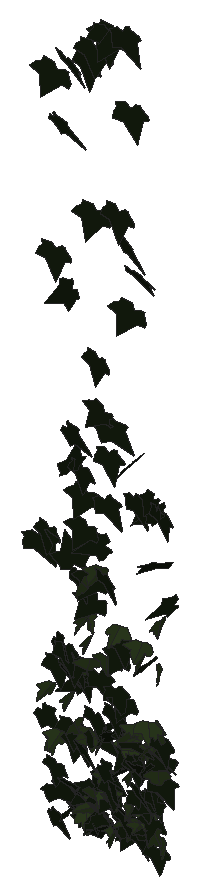
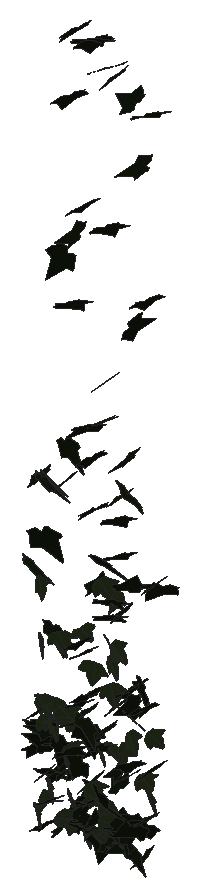
# SketchUp Ruby script. Lengths in inches.
U = 1.inch
M = Sketchup.active_model
def pt(a) = Geom::Point3d.new(a.map { |v| v * U })
def face(e, loops, mat)
  f = e.add_face(loops[0].map { |a| pt(a) })
  loops[1..].each { |l| e.add_face(l.map { |a| pt(a) }).erase! }
  f.material = f.back_material = mat if mat
  f
end
# faces: each face lists its corners as indices into pts; further lists are holes
def faces(e, pts, list, mat = nil) = list.each { |f| face(e, (f[0].is_a?(Array) ? f : [f]).map { |l| l.map { |i| pts[i] } }, mat) }
# xy, xz, yz: faces in a plane at the given z, y or x. An outline is a flat list of corners, or four numbers for a rectangle; further outlines are holes
def ring(l) = l.size == 4 ? [[l[0], l[1]], [l[2], l[1]], [l[2], l[3]], [l[0], l[3]]] : l.each_slice(2).to_a
def flat(e, list, mat, &to3) = list.each { |f| face(e, (f[0].is_a?(Array) ? f : [f]).map { |l| ring(l).map { |u, v| to3.(u, v) } }, mat) }
def xy(e, z, list, mat = nil) = flat(e, list, mat) { |x, y| [x, y, z] }
def xz(e, y, list, mat = nil) = flat(e, list, mat) { |x, z| [x, y, z] }
def yz(e, x, list, mat = nil) = flat(e, list, mat) { |y, z| [x, y, z] }
def lines(e, pts, list) = list.each { |a, b| e.add_line(pt(pts[a]), pt(pts[b])) }
# prism: a flat outline (further loops are holes) pulled along v
def prism(e, loops, v, mat = nil)
  f = face(e, loops, mat); d = Geom::Vector3d.new(v.map { |x| x * U })
  f.pushpull(f.normal.samedirection?(d) ? d.length : -d.length)
end
def box(e, o, s, mat = nil) = prism(e, [[o, [o[0] + s[0], o[1], o[2]], [o[0] + s[0], o[1] + s[1], o[2]], [o[0], o[1] + s[1], o[2]]]], [0, 0, s[2]], mat)
def at(x, y, z, deg = 0) = Geom::Transformation.translation(pt([x, y, z])) * Geom::Transformation.rotation(ORIGIN, Z_AXIS, deg.degrees)
def axes(o, x, y, z) = Geom::Transformation.new([*x, 0, *y, 0, *z, 0, *pt(o).to_a, 1])
def part(name) = M.definitions.add(name)
# library, detail: a bought-in or finely detailed component or shape, given as its bounding box
def library(name, o, s) = part(name).tap { |d| box(d.entities, o, s) }
def detail(e, o, s) = box(e.add_group.entities, o, s)
def put(e, d, t, mat = nil) = e.add_instance(d, t).tap { |i| i.material = mat if mat }
def group(e, t, mat = nil) = e.add_group.tap { |g| g.transformation = t; g.material = mat if mat }.entities
root = M.entities
M.materials.add("1026 AP 7946 SUNNY SIDE UP").color = [254, 231, 186]
M.materials.add("efeu1").color = [18, 25, 13]
M.materials.add("efeu2").color = [43, 57, 29]
c1 = part("ivyleaf_10")
p = [[0,0.5,-0.03],[-0.0625,2.02,-0.43],[-0.19,2.01,-0.46],[-0.54,1.05,-0.29],[-0.52,0.625,-0.18],[-0.83,0.76,-0.28],
  [-1.16,0.64,-0.33],[-1.15,0.33,-0.24],[-0.77,-0.39,0.02],[-0.3,-0.51,0.16],[0.04,-0.48,0.23],[-0.02,2.01,-0.4375],
  [-0.06,2.01,-0.43],[0.04,-0.49,0.23],[0.67,-0.49,0.14],[1.38,0.36,-0.2],[1.375,0.51,-0.24],[0.81,0.65,-0.19],
  [0.62,0.59,-0.15],[0.6,1.09,-0.28],[0.5,1.23,-0.31]]
faces(c1.entities,p,[[0,1,2,3,4,5,6,7,8,9,10],[11,12,0,13,14,15,16,17,18,19,20]],"efeu2")
c2 = part("ivyleaf_9")
p = [[1.54,2.16,1.25],[1.36,2.04,1.19],[-0.21,0.99,0.68],[-0.71,1.11,0.82],[-0.85,0.86,0.67],[-0.8,0.17,0.21],
  [-0.9,-0.01,0.1],[-0.67,-0.16,-0.02],[-0.08,-0.08,-0.05],[-0.03,-0.6,-0.4],[0.65,-0.88,-0.66],[0.83,-0.6,-0.49],
  [1.29,-0.42,-0.43],[1.8125,-0.07,-0.26],[1.21,0.44,0.15]]
faces(c2.entities,p,[[0,1,2,3,4,5,6,7,8,9,10,11,12,13,14]],"efeu1")
put(root,c1,axes([134.13,212.53,294.28],[0.33293,-0.26195,-0.18887],[-0.15797,0.15237,-0.34573],[0.47588,0.23384,0.01737]),"1026 AP 7946 SUNNY SIDE UP")
put(root,c2,axes([133.74,212.17,304.24],[-0.13472,-0.32165,-0.27255],[0.20303,0.23434,-0.33756],[0.62068,-0.14647,0.05126]),"1026 AP 7946 SUNNY SIDE UP")
put(root,c2,axes([133.88,212.625,304.42],[-0.05844,-0.37294,0.13765],[-0.03565,-0.13411,-0.38678],[0.62303,-0.04265,-0.00922]),"1026 AP 7946 SUNNY SIDE UP")
put(root,c1,axes([134.12,212.36,297.02],[-0.10301,-0.29039,0.23968],[-0.02573,-0.23542,-0.30668],[0.58614,-0.06137,0.02866]),"1026 AP 7946 SUNNY SIDE UP")
put(root,c2,axes([133.82,212.36,295.7],[0.26681,-0.28497,-0.23819],[-0.09029,0.2292,-0.33545],[0.56828,0.17021,0.05853]),"1026 AP 7946 SUNNY SIDE UP")
put(root,c2,axes([134.19,212.69,318.03],[-0.1405,-0.4347,0.0012],[0.00417,-0.00426,-0.4572],[0.68354,-0.08933,0.00304]),"1026 AP 7946 SUNNY SIDE UP")
put(root,c2,axes([134.34,212.52,326.82],[-0.41289,-0.37471,0.12809],[0.01519,-0.15783,-0.46204],[0.62165,-0.24502,0.09636]),"1026 AP 7946 SUNNY SIDE UP")
put(root,c2,axes([134.22,212.72,293.07],[-0.08881,-0.32549,0.15097],[0.04328,-0.15374,-0.33751],[0.56082,-0.03968,0.04996]),"1026 AP 7946 SUNNY SIDE UP")
put(root,c1,axes([134.59,212.38,294.82],[-0.24139,-0.27422,0.22648],[0.0221,-0.24606,-0.30537],[0.55374,-0.10972,0.11092]),"1026 AP 7946 SUNNY SIDE UP")
put(root,c2,axes([134.48,212.51,298.29],[-0.08486,-0.39007,-0.02198],[0.0001,0.0193,-0.40555],[0.61408,-0.0539,-0.00297]),"1026 AP 7946 SUNNY SIDE UP")
put(root,c2,axes([134.35,212.6,299.22],[0.02918,-0.12609,-0.38308],[0.60824,-0.05416,0.03857],[-0.09961,-0.36764,0.12325]),"1026 AP 7946 SUNNY SIDE UP")
put(root,c2,axes([134.34,212.58,324.43],[0.52513,-0.31138,-0.06126],[0.01397,0.09304,-0.46371],[0.49775,0.32589,0.07765]),"1026 AP 7946 SUNNY SIDE UP")
put(root,c2,axes([134.53,212.125,291.1],[0.32327,-0.27561,-0.11867],[-0.10007,0.09427,-0.35363],[0.45795,0.21516,0.00649]),"1026 AP 7946 SUNNY SIDE UP")
put(root,c2,axes([135.16,212.43,291.24],[-0.21083,0.3254,-0.01468],[-0.00983,-0.01997,-0.36243],[-0.5122,-0.13356,0.013]),"1026 AP 7946 SUNNY SIDE UP")
put(root,c2,axes([134.62,212.15,292.4375],[0.03625,-0.139,-0.36574],[0.18005,0.34096,-0.12817],[0.57061,-0.09876,0.06368]),"1026 AP 7946 SUNNY SIDE UP")
put(root,c1,axes([135.04,212.625,296.77],[-0.00007,-0.38183,0.03941],[-0.00016,-0.04043,-0.39359],[0.60374,-0.00006,-0.0001]),"1026 AP 7946 SUNNY SIDE UP")
put(root,c2,axes([135.05,212.62,316.4375],[0.00082,-0.21928,-0.43947],[0.28433,-0.39372,0.20703],[-0.69667,-0.16094,0.08398]),"1026 AP 7946 SUNNY SIDE UP")
put(root,c2,axes([134.74,212.4,292.5],[0.56784,0.02559,0.08434],[0.13176,-0.03258,-0.37115],[-0.02776,0.36882,-0.03645]),"1026 AP 7946 SUNNY SIDE UP")
put(root,c2,axes([134.73,212.79,327.375],[0.22262,-0.37505,0.24704],[0.18751,-0.21279,-0.41298],[0.67626,0.18246,0.03319]),"1026 AP 7946 SUNNY SIDE UP")
put(root,c2,axes([135,212.37,299.14],[0.02752,-0.39373,-0.01249],[-0.00676,0.0097,-0.40594],[0.61926,0.0176,-0.00388]),"1026 AP 7946 SUNNY SIDE UP")
put(root,c2,axes([135.4,212.24,308.1],[-0.50944,0.28383,-0.19066],[-0.18303,0.14961,0.44332],[0.50185,0.34269,-0.03187]),"1026 AP 7946 SUNNY SIDE UP")
put(root,c2,axes([135.17,212.625,295.42],[-0.17406,-0.35467,-0.0606],[0.03547,0.05247,-0.38241],[0.56368,-0.11282,0.00535]),"1026 AP 7946 SUNNY SIDE UP")
put(root,c2,axes([135.53,212.24,303.56],[-0.54205,-0.18855,0.16931],[0.20464,0.1059,0.40437],[-0.33716,0.3674,-0.02678]),"1026 AP 7946 SUNNY SIDE UP")
put(root,c2,axes([134.98,212.29,298.13],[0.51508,-0.19503,0.03846],[0.02793,-0.04508,-0.39183],[0.31131,0.32673,-0.02848]),"1026 AP 7946 SUNNY SIDE UP")
put(root,c2,axes([135.33,212.66,294.73],[-0.11052,-0.34686,0.12552],[0.00577,-0.1267,-0.36426],[0.57907,-0.06494,0.02758]),"1026 AP 7946 SUNNY SIDE UP")
put(root,c2,axes([135.87,212.41,297.84],[-0.54011,0.17301,0.01063],[-0.03987,-0.02969,-0.39446],[-0.26951,-0.34233,0.03705]),"1026 AP 7946 SUNNY SIDE UP")
put(root,c2,axes([135.22,212.48,291.52],[0.49824,-0.18281,0.01197],[0.01835,-0.0051,-0.37689],[0.28755,0.31708,0.00331]),"1026 AP 7946 SUNNY SIDE UP")
put(root,c2,axes([135.45,212.4375,298.71],[-0.11702,-0.38131,0.0361],[-0.00021,-0.03788,-0.40039],[0.60242,-0.07408,0.00688]),"1026 AP 7946 SUNNY SIDE UP")
put(root,c2,axes([135.33,212.16,309.95],[0.40059,-0.29519,-0.18227],[-0.10396,0.17197,-0.3964],[0.52969,0.257,0.06005]),"1026 AP 7946 SUNNY SIDE UP")
put(root,c2,axes([135.39,212.76,302.66],[0.12527,-0.38162,0.07901],[0.00832,-0.07942,-0.40193],[0.61268,0.0791,-0.01069]),"1026 AP 7946 SUNNY SIDE UP")
put(root,c1,axes([135.71,212.12,295.8125],[-0.11454,-0.3205,-0.20139],[0.11258,0.18173,-0.33652],[0.57795,-0.09892,0.02564]),"1026 AP 7946 SUNNY SIDE UP")
put(root,c1,axes([135.83,212.62,300.75],[0.02841,-0.36397,0.1611],[-0.0157,-0.15898,-0.37598],[0.62399,0.01257,-0.0168]),"1026 AP 7946 SUNNY SIDE UP")
put(root,c2,axes([135.54,212.73,294.27],[0.04237,-0.25488,0.26857],[0.15172,-0.24858,-0.26066],[0.55454,0.08749,0.0508]),"1026 AP 7946 SUNNY SIDE UP")
put(root,c2,axes([135.84,212.68,305.18],[-0.33757,-0.32453,0.11841],[-0.02098,-0.12964,-0.39717],[0.54193,-0.20717,0.05838]),"1026 AP 7946 SUNNY SIDE UP")
put(root,c2,axes([135.7,212.61,307.96],[-0.038,-0.37972,0.16198],[0.02841,-0.16048,-0.392],[0.64691,-0.01526,0.02673]),"1026 AP 7946 SUNNY SIDE UP")
put(root,c2,axes([135.95,212.58,306.87],[-0.36768,-0.3281,0.05341],[-0.00843,-0.06193,-0.41417],[0.5227,-0.23179,0.03089]),"1026 AP 7946 SUNNY SIDE UP")
put(root,c1,axes([136.0625,212.64,298.74],[-0.37255,-0.30325,0.0503],[-0.01619,-0.05595,-0.39586],[0.48314,-0.23571,0.02552]),"1026 AP 7946 SUNNY SIDE UP")
put(root,c2,axes([135.78,212.65,297.97],[0.0469,-0.37594,0.07841],[0.01126,-0.07792,-0.38896],[0.60369,0.03066,0.00117]),"1026 AP 7946 SUNNY SIDE UP")
put(root,c2,axes([136.4,212.21,291.54],[-0.28359,0.29837,0.11667],[-0.13408,0.0783,-0.35729],[-0.48259,-0.19709,0.03071]),"1026 AP 7946 SUNNY SIDE UP")
put(root,c1,axes([136.16,212.53,299.97],[0.05495,-0.38936,0.04866],[0.00257,-0.04949,-0.403],[0.61714,0.03487,-0.00266]),"1026 AP 7946 SUNNY SIDE UP")
put(root,c2,axes([135.83,212.27,294.79],[0.3657,-0.29299,0.00758],[-0.01187,-0.0175,-0.38509],[0.46077,0.23209,-0.01594]),"1026 AP 7946 SUNNY SIDE UP")
put(root,c2,axes([136.37,212.39,292.73],[-0.57597,0.03668,-0.04625],[0.06558,-0.03463,-0.37818],[-0.06368,-0.36743,0.02883]),"1026 AP 7946 SUNNY SIDE UP")
put(root,c1,axes([135.99,212.79,300.8],[-0.20193,0.06362,-0.3742],[0.18322,-0.3583,-0.10908],[-0.55073,-0.14253,0.10091]),"1026 AP 7946 SUNNY SIDE UP")
put(root,c2,axes([135.77,212.36,292.26],[0.22882,-0.2253,0.24102],[0.26885,-0.16645,-0.27418],[0.43593,0.22092,0.04258]),"1026 AP 7946 SUNNY SIDE UP")
put(root,c2,axes([136.36,212.67,302.85],[-0.48518,-0.24765,0.03921],[0.03202,-0.08712,-0.39963],[0.39301,-0.29863,0.08096]),"1026 AP 7946 SUNNY SIDE UP")
put(root,c1,axes([136.25,211.97,302.85],[-0.03853,-0.3051,-0.271],[0.13975,0.2512,-0.30926],[0.61601,-0.07607,0.05321]),"1026 AP 7946 SUNNY SIDE UP")
put(root,c1,axes([136.56,212.11,295.52],[0.38087,-0.16405,-0.27905],[-0.37835,0.12457,-0.29969],[0.3218,0.34062,-0.02208]),"1026 AP 7946 SUNNY SIDE UP")
put(root,c1,axes([136.57,212.39,292.05],[-0.10041,-0.11932,0.37402],[-0.25664,-0.32508,-0.14128],[0.54447,-0.17523,0.00238]),"1026 AP 7946 SUNNY SIDE UP")
put(root,c2,axes([136.08,212.49,327.94],[0.02669,-0.44324,0.16773],[-0.00194,-0.16548,-0.45786],[0.74385,0.01547,-0.00721]),"1026 AP 7946 SUNNY SIDE UP")
put(root,c1,axes([136.28,212.16,291.59],[0.35256,0.31824,-0.01211],[0.01599,-0.02372,-0.40055],[-0.50061,0.22337,-0.02132]),"1026 AP 7946 SUNNY SIDE UP")
put(root,c2,axes([136.53,212.49,301.96],[-0.47063,-0.24398,0.1062],[-0.04285,-0.12838,-0.39005],[0.41513,-0.28986,0.08013]),"1026 AP 7946 SUNNY SIDE UP")
put(root,c2,axes([136.23,212.75,291.22],[0.02286,-0.2588,0.25092],[0.07664,-0.24149,-0.26715],[0.55514,0.044,0.02655]),"1026 AP 7946 SUNNY SIDE UP")
put(root,c2,axes([136.875,212.6,304.65],[-0.59071,0.10779,0.09674],[-0.15669,-0.01054,-0.40093],[-0.16029,-0.38694,0.03543]),"1026 AP 7946 SUNNY SIDE UP")
put(root,c2,axes([136.33,212.85,313.39],[-0.0578,-0.39538,0.15563],[-0.01603,-0.15302,-0.40995],[0.66661,-0.03796,0.00364]),"1026 AP 7946 SUNNY SIDE UP")
put(root,c2,axes([136.46,212.55,320.69],[-0.34014,-0.3937,0.03817],[-0.00661,-0.04249,-0.46271],[0.6221,-0.21571,0.01595]),"1026 AP 7946 SUNNY SIDE UP")
put(root,c2,axes([136.31,212.75,328.47],[-0.20883,-0.44222,0.09624],[0.12558,-0.12132,-0.46293],[0.70035,-0.11011,0.11171]),"1026 AP 7946 SUNNY SIDE UP")
put(root,c1,axes([136.72,212.48,303.46],[-0.25504,-0.30698,0.20112],[-0.07127,-0.19693,-0.35579],[0.56907,-0.16224,0.04558]),"1026 AP 7946 SUNNY SIDE UP")
put(root,c2,axes([136.68,212.45,291.7],[-0.46589,-0.19518,-0.03706],[0.06165,0.00377,-0.365],[0.3056,-0.29831,0.01714]),"1026 AP 7946 SUNNY SIDE UP")
put(root,c1,axes([136.79,212.16,292.8125],[-0.56836,0.04586,0.01624],[-0.03149,-0.03535,-0.37356],[-0.06929,-0.36006,0.03658]),"1026 AP 7946 SUNNY SIDE UP")
put(root,c2,axes([136.79,212.19,291.0625],[0.25093,0.31526,-0.00249],[-0.0068,-0.00253,-0.36402],[-0.49571,0.15962,0.00373]),"1026 AP 7946 SUNNY SIDE UP")
put(root,c2,axes([136.54,212.4,296.42],[0.0569,-0.3569,0.12605],[0.03626,-0.12263,-0.37014],[0.59319,0.04173,0.01053]),"1026 AP 7946 SUNNY SIDE UP")
put(root,c2,axes([136.85,212.57,311.15],[-0.34421,-0.26374,0.25388],[-0.04355,-0.2767,-0.33003],[0.56751,-0.1812,0.12866]),"1026 AP 7946 SUNNY SIDE UP")
put(root,c1,axes([136.96,212.35,295.42],[0.24511,-0.34259,0.01472],[-0.00041,-0.01795,-0.38777],[0.53929,0.1557,-0.00699]),"1026 AP 7946 SUNNY SIDE UP")
put(root,c1,axes([137.21,212.4375,291.4],[0.35476,-0.09871,-0.26575],[-0.38852,0.0751,-0.25234],[0.19223,0.33394,-0.01958]),"1026 AP 7946 SUNNY SIDE UP")
put(root,c2,axes([136.7,212.33,295.625],[0.11868,-0.27701,-0.25064],[0.07347,0.25198,-0.28099],[0.5734,0.02504,0.08788]),"1026 AP 7946 SUNNY SIDE UP")
put(root,c1,axes([137.07,212.63,293.68],[-0.24529,-0.31447,0.12547],[-0.0089,-0.13367,-0.35854],[0.53121,-0.14745,0.05193]),"1026 AP 7946 SUNNY SIDE UP")
put(root,c2,axes([136.79,212.4,298.43],[0.06306,-0.36889,-0.10843],[0.04578,0.10636,-0.37953],[0.60055,0.03063,0.04032]),"1026 AP 7946 SUNNY SIDE UP")
put(root,c1,axes([137.22,212.44,299.32],[-0.60972,-0.00057,0.0415],[-0.06306,-0.03156,-0.39835],[0.00602,-0.38857,0.03001]),"1026 AP 7946 SUNNY SIDE UP")
put(root,c2,axes([136.79,212.64,293.53],[-0.18257,-0.09175,-0.40902],[0.62206,0.07138,-0.13594],[0.15027,-0.40695,0.0658]),"1026 AP 7946 SUNNY SIDE UP")
put(root,c2,axes([137.07,212.69,329.51],[-0.1857,-0.46035,-0.05156],[0.01281,0.04688,-0.48931],[0.72757,-0.11832,-0.00454]),"1026 AP 7946 SUNNY SIDE UP")
put(root,c2,axes([137,212.4,294.08],[0.33086,-0.24007,-0.20567],[-0.12871,0.18824,-0.32318],[0.47236,0.21944,0.05599]),"1026 AP 7946 SUNNY SIDE UP")
put(root,c2,axes([137.28,212.77,329.5],[-0.49707,-0.34834,0.06188],[0.06103,-0.11684,-0.47274],[0.55299,-0.30022,0.1078]),"1026 AP 7946 SUNNY SIDE UP")
put(root,c2,axes([137.02,212.42,303.29],[0.20541,-0.35631,0.12053],[0.04863,-0.11539,-0.3915],[0.58869,0.13386,-0.00971]),"1026 AP 7946 SUNNY SIDE UP")
put(root,c2,axes([137.37,212.54,292.8],[-0.28172,-0.28217,0.14399],[-0.06028,-0.14191,-0.34266],[0.49259,-0.17875,0.04042]),"1026 AP 7946 SUNNY SIDE UP")
put(root,c2,axes([137.09,212.45,306.95],[0.11267,-0.38415,-0.13889],[0.04148,0.1388,-0.39863],[0.63769,0.05884,0.05047]),"1026 AP 7946 SUNNY SIDE UP")
put(root,c1,axes([137.25,212.22,292.88],[0.26395,0.31527,0.15865],[0.14492,0.12305,-0.36656],[-0.53106,0.19027,-0.02118]),"1026 AP 7946 SUNNY SIDE UP")
put(root,c2,axes([137.33,212.63,293.2],[-0.08629,-0.36784,-0.00128],[-0.00367,-0.00051,-0.38314],[0.57839,-0.05488,-0.00262]),"1026 AP 7946 SUNNY SIDE UP")
put(root,c2,axes([137.75,212.29,296.45],[-0.10631,0.38537,0.09939],[-0.05382,0.08962,-0.40213],[-0.6215,-0.07368,0.01783]),"1026 AP 7946 SUNNY SIDE UP")
put(root,c2,axes([137.3,212.43,309.31],[-0.02909,-0.42417,-0.04187],[-0.00803,0.03849,-0.43711],[0.66961,-0.01796,-0.00706]),"1026 AP 7946 SUNNY SIDE UP")
put(root,c2,axes([137.64,212.18,296.06],[0.11372,0.37347,-0.11558],[-0.03514,-0.11211,-0.39255],[-0.61314,0.0757,0.00106]),"1026 AP 7946 SUNNY SIDE UP")
put(root,c2,axes([137.23,212.37,291.72],[0.22739,-0.26103,0.21101],[0.12446,-0.19151,-0.30789],[0.50814,0.16371,-0.01901]),"1026 AP 7946 SUNNY SIDE UP")
put(root,c1,axes([137.75,212.48,300.93],[0.29229,0.29128,-0.19977],[-0.17668,-0.16023,-0.35683],[-0.5226,0.21708,0.00891]),"1026 AP 7946 SUNNY SIDE UP")
put(root,c1,axes([137.77,212.19,291.18],[0.07918,-0.36216,-0.01381],[-0.00278,0.01121,-0.37662],[0.56974,0.05039,0.00008]),"1026 AP 7946 SUNNY SIDE UP")
put(root,c2,axes([137.55,212.58,297.86],[0.0121,-0.36241,-0.11236],[-0.01845,0.10675,-0.37269],[0.59389,0.0107,-0.00929]),"1026 AP 7946 SUNNY SIDE UP")
put(root,c2,axes([137.41,212.33,310.72],[0.13611,-0.33032,-0.26127],[0.10904,0.26503,-0.33215],[0.64386,0.02494,0.11148]),"1026 AP 7946 SUNNY SIDE UP")
put(root,c2,axes([137.48,212.61,292.28],[0.50687,-0.16244,0.01644],[0.00074,-0.03642,-0.37059],[0.2568,0.32073,-0.03138]),"1026 AP 7946 SUNNY SIDE UP")
put(root,c2,axes([137.64,212.39,296.92],[0.01101,-0.36292,0.13642],[0.04221,-0.13373,-0.37399],[0.6071,0.01588,0.02353]),"1026 AP 7946 SUNNY SIDE UP")
put(root,c2,axes([137.84,212.51,299.73],[-0.23553,-0.30074,0.18813],[-0.05115,-0.18763,-0.34369],[0.55227,-0.14563,0.0484]),"1026 AP 7946 SUNNY SIDE UP")
put(root,c2,axes([137.89,212.82,297.42],[-0.26341,-0.32009,0.11551],[0.0051,-0.12854,-0.36784],[0.53423,-0.1566,0.06046]),"1026 AP 7946 SUNNY SIDE UP")
put(root,c2,axes([137.81,212.46,321.19],[-0.1006,-0.45101,0.07334],[-0.00088,-0.0744,-0.4696],[0.71859,-0.06323,0.00969]),"1026 AP 7946 SUNNY SIDE UP")
put(root,c2,axes([137.84,212.72,300.35],[-0.08395,-0.38844,0.018],[0.00348,-0.02017,-0.40402],[0.61156,-0.05321,0.00477]),"1026 AP 7946 SUNNY SIDE UP")
put(root,c2,axes([138.04,212.2,294.32],[0.17934,0.29336,0.24068],[0.14791,0.21221,-0.32289],[-0.56916,0.14759,-0.00807]),"1026 AP 7946 SUNNY SIDE UP")
put(root,c2,axes([138.28,212.9,295.06],[-0.375,-0.30896,0.17815],[-0.13742,-0.15286,-0.40233],[0.5409,-0.25303,0.0213]),"1026 AP 7946 SUNNY SIDE UP")
put(root,c1,axes([138.22,212.59,291.74],[-0.34575,-0.28242,-0.03422],[0.09598,-0.0079,-0.36474],[0.43642,-0.22201,0.0531]),"1026 AP 7946 SUNNY SIDE UP")
put(root,c2,axes([137.92,212.63,329.8125],[0.14439,-0.44432,-0.14592],[0.00128,0.14195,-0.46568],[0.7321,0.08739,0.02959]),"1026 AP 7946 SUNNY SIDE UP")
put(root,c1,axes([138.09,212.78,295.4],[-0.31825,-0.2779,0.18618],[0.26864,-0.27008,-0.23031],[0.44827,-0.03544,0.2702]),"1026 AP 7946 SUNNY SIDE UP")
put(root,c2,axes([138.32,212.73,316.49],[-0.42925,-0.33529,0.08038],[-0.02282,-0.09069,-0.4435],[0.5415,-0.2696,0.04503]),"1026 AP 7946 SUNNY SIDE UP")
put(root,c2,axes([138.05,212.55,291.94],[-0.04506,-0.31305,0.19557],[0.1432,-0.19226,-0.31067],[0.55908,0.02401,0.09534]),"1026 AP 7946 SUNNY SIDE UP")
put(root,c2,axes([138.4,212.76,291.72],[-0.48267,-0.18311,0.02982],[0.04792,-0.10694,-0.35194],[0.2878,-0.28929,0.10862]),"1026 AP 7946 SUNNY SIDE UP")
put(root,c2,axes([138.375,212.71,291.46],[-0.46655,-0.20423,-0.05886],[0.13931,-0.03221,-0.36295],[0.30243,-0.30022,0.07639]),"1026 AP 7946 SUNNY SIDE UP")
put(root,c2,axes([137.97,212.49,319.85],[0.44588,-0.37452,0.01272],[-0.00019,-0.01825,-0.48392],[0.58934,0.28335,-0.00979]),"1026 AP 7946 SUNNY SIDE UP")
put(root,c1,axes([138.39,212.64,294.44],[0.21774,-0.3479,-0.01258],[0.00385,0.01199,-0.38561],[0.54725,0.13833,0.00772]),"1026 AP 7946 SUNNY SIDE UP")
put(root,c1,axes([138.43,212.42,292.64],[0.34713,-0.29495,-0.00039],[0.00563,0.00105,-0.37952],[0.46374,0.22077,0.00489]),"1026 AP 7946 SUNNY SIDE UP")
put(root,c2,axes([138.69,212.34,309.47],[-0.24457,0.36846,-0.15584],[0.09213,-0.14173,-0.41284],[-0.62075,-0.1662,0.00013]),"1026 AP 7946 SUNNY SIDE UP")
put(root,c1,axes([138.7,212.59,291.71],[-0.1892,-0.27931,0.19721],[-0.03956,-0.19688,-0.31081],[0.53238,-0.11389,0.04699]),"1026 AP 7946 SUNNY SIDE UP")
put(root,c2,axes([138.4,212.53,326.33],[-0.08535,-0.45279,-0.09588],[0.01887,0.08971,-0.46928],[0.72581,-0.05558,0.00093]),"1026 AP 7946 SUNNY SIDE UP")
put(root,c1,axes([138.72,212.24,294.51],[0.03131,-0.39181,-0.02218],[-0.01338,0.01889,-0.40398],[0.61669,0.02031,-0.00764]),"1026 AP 7946 SUNNY SIDE UP")
put(root,c1,axes([138.77,212.76,300.39],[-0.42264,-0.24563,0.14436],[0.00834,-0.19935,-0.34722],[0.44567,-0.2292,0.1434]),"1026 AP 7946 SUNNY SIDE UP")
put(root,c1,axes([138.52,211.91,295.98],[0.01982,-0.10985,0.38453],[0.15345,0.36305,0.10862],[-0.59322,0.09024,0.04094]),"1026 AP 7946 SUNNY SIDE UP")
put(root,c1,axes([138.89,212.32,296.54],[-0.33123,-0.20865,0.24573],[-0.10251,-0.2531,-0.28746],[0.48908,-0.19436,0.10617]),"1026 AP 7946 SUNNY SIDE UP")
put(root,c2,axes([138.34,212.18,296.125],[0.29496,-0.3422,-0.05992],[0.26416,0.14559,-0.33461],[0.47704,0.13097,0.22234]),"1026 AP 7946 SUNNY SIDE UP")
put(root,c2,axes([138.64,212.54,294.8125],[-0.00754,-0.36039,0.05547],[0.00754,-0.05596,-0.37159],[0.57341,-0.004,0.00562]),"1026 AP 7946 SUNNY SIDE UP")
put(root,c2,axes([138.59,212.73,291.24],[0.17332,-0.34155,0.04272],[0.01252,-0.04303,-0.36994],[0.54123,0.11037,-0.00512]),"1026 AP 7946 SUNNY SIDE UP")
put(root,c2,axes([138.7,212.4,318.57],[0.66595,-0.02196,-0.1632],[-0.2454,0.03957,-0.43561],[0.05403,0.4504,0.03297]),"1026 AP 7946 SUNNY SIDE UP")
put(root,c2,axes([138.93,212.12,294.9],[0.5066,0.08972,-0.17342],[-0.24139,-0.07583,-0.34374],[-0.17922,0.35575,-0.02722]),"1026 AP 7946 SUNNY SIDE UP")
put(root,c1,axes([138.97,212.52,299.96],[0.2133,-0.35394,0.10426],[0.03061,-0.10295,-0.39065],[0.5789,0.13585,-0.01776]),"1026 AP 7946 SUNNY SIDE UP")
put(root,c2,axes([138.73,212.34,307.67],[0.20148,-0.39134,-0.04498],[-0.02525,0.03834,-0.42398],[0.61827,0.12909,-0.00266]),"1026 AP 7946 SUNNY SIDE UP")
put(root,c2,axes([138.88,212.26,293.75],[0.35424,-0.29688,0.02995],[-0.00047,-0.03877,-0.38339],[0.46932,0.22405,-0.02299]),"1026 AP 7946 SUNNY SIDE UP")
put(root,c1,axes([139.07,212.78,292.32],[-0.43016,-0.19631,0.16659],[0.26264,-0.31835,-0.10816],[0.30307,-0.00276,0.33018]),"1026 AP 7946 SUNNY SIDE UP")
put(root,c2,axes([139.39,212.68,307.71],[-0.57247,0.04973,-0.19025],[0.26324,-0.11035,-0.37069],[-0.14628,-0.39317,0.07746]),"1026 AP 7946 SUNNY SIDE UP")
put(root,c2,axes([139.08,212.26,293.49],[-0.01073,-0.35974,-0.10152],[0.04605,0.0957,-0.3691],[0.58384,-0.01416,0.02724]),"1026 AP 7946 SUNNY SIDE UP")
put(root,c1,axes([139.46,212.37,295.82],[0.05525,-0.38035,-0.01088],[-0.01721,0.00742,-0.39332],[0.59796,0.03535,-0.01031]),"1026 AP 7946 SUNNY SIDE UP")
put(root,c2,axes([139.69,211.95,300.08],[-0.11811,0.3952,0.06843],[-0.04015,0.06043,-0.41383],[-0.62827,-0.07816,0.01358]),"1026 AP 7946 SUNNY SIDE UP")
put(root,c2,axes([139.83,212.52,304.83],[-0.03023,0.34974,-0.21958],[-0.17605,-0.21168,-0.34544],[-0.62118,0.04297,0.10859]),"1026 AP 7946 SUNNY SIDE UP")
put(root,c2,axes([139.52,212.72,292.17],[-0.21415,-0.32118,0.10857],[0.00238,-0.11614,-0.35711],[0.53241,-0.12867,0.04527]),"1026 AP 7946 SUNNY SIDE UP")
put(root,c1,axes([139.68,212.57,295.97],[-0.23472,-0.32314,0.14296],[-0.00116,-0.15241,-0.36255],[0.55412,-0.1372,0.05979]),"1026 AP 7946 SUNNY SIDE UP")
put(root,c2,axes([139.84,212.39,293.39],[-0.54078,-0.11513,0.08885],[-0.08664,-0.10278,-0.36554],[0.20961,-0.33951,0.07813]),"1026 AP 7946 SUNNY SIDE UP")
put(root,c1,axes([140.03,212.48,296.66],[-0.17744,0.12465,0.35582],[-0.5459,0.07929,-0.14617],[-0.1848,-0.35391,0.09014]),"1026 AP 7946 SUNNY SIDE UP")
put(root,c1,axes([139.45,212.34,296.91],[0.5628,0.13267,0.07569],[0.12422,-0.00459,-0.39196],[-0.20289,0.36521,-0.03001]),"1026 AP 7946 SUNNY SIDE UP")
put(root,c2,axes([139.99,212.44,307.41],[-0.54678,0.22563,-0.07513],[0.01304,-0.11995,-0.41647],[-0.37324,-0.33472,0.0955]),"1026 AP 7946 SUNNY SIDE UP")
put(root,c1,axes([139.77,212.17,292.68],[0.16451,-0.30568,-0.17473],[-0.08053,0.1599,-0.3319],[0.54242,0.11645,0.00372]),"1026 AP 7946 SUNNY SIDE UP")
put(root,c2,axes([139.57,212.62,293.49],[0.10339,-0.35894,0.0315],[-0.01409,-0.03477,-0.37582],[0.56655,0.06464,-0.01509]),"1026 AP 7946 SUNNY SIDE UP")
put(root,c2,axes([139.45,212.54,295.6],[0.38944,-0.22463,0.15608],[0.20503,-0.08307,-0.34408],[0.37474,0.2789,0.02606]),"1026 AP 7946 SUNNY SIDE UP")
put(root,c2,axes([139.74,212.63,290.93],[-0.06651,-0.35592,-0.00518],[0.01912,0.00159,-0.36903],[0.55934,-0.04238,0.012]),"1026 AP 7946 SUNNY SIDE UP")
put(root,c1,axes([139.98,212.47,299.71],[0.25715,-0.32525,-0.14755],[-0.02132,0.14984,-0.3704],[0.55724,0.15582,0.05392]),"1026 AP 7946 SUNNY SIDE UP")
put(root,c2,axes([139.74,212.15,294.64],[0.03078,0.01953,0.40343],[0.53413,0.19475,-0.02637],[-0.30756,0.34018,-0.00541]),"1026 AP 7946 SUNNY SIDE UP")
put(root,c2,axes([140.31,212.56,295.61],[-0.57182,-0.09575,0.06399],[-0.08264,-0.04567,-0.38641],[0.15983,-0.36618,0.02914]),"1026 AP 7946 SUNNY SIDE UP")
put(root,c1,axes([140.15,212.2,294.9],[-0.39515,-0.268,0.00683],[0.01771,-0.02171,-0.37786],[0.42122,-0.2505,0.02229]),"1026 AP 7946 SUNNY SIDE UP")
put(root,c1,axes([140.1,212.04,291.97],[-0.01759,-0.31893,-0.19541],[0.11102,0.18267,-0.32272],[0.57135,-0.04531,0.0567]),"1026 AP 7946 SUNNY SIDE UP")
put(root,c1,axes([140.28,212.38,291.4375],[0.25325,-0.27091,-0.1986],[-0.10074,0.18318,-0.32184],[0.5116,0.17018,0.03493]),"1026 AP 7946 SUNNY SIDE UP")
put(root,c1,axes([140.21,212.22,302.28],[-0.00847,-0.40198,-0.00879],[0.05854,0.00573,-0.41235],[0.62944,-0.00594,0.03823]),"1026 AP 7946 SUNNY SIDE UP")
put(root,c2,axes([140.03,212.59,296.27],[0.02017,-0.38122,0.03999],[-0.00704,-0.04115,-0.39315],[0.60285,0.01227,-0.00593]),"1026 AP 7946 SUNNY SIDE UP")
put(root,c2,axes([140.06,212.46,307.39],[0.09783,-0.38638,0.15958],[0.04484,-0.15452,-0.40406],[0.6543,0.06836,0.00383]),"1026 AP 7946 SUNNY SIDE UP")
put(root,c2,axes([140.125,212.43,294.47],[-0.05751,-0.3331,-0.17567],[0.09258,0.16217,-0.34222],[0.57972,-0.05895,0.03722]),"1026 AP 7946 SUNNY SIDE UP")
put(root,c2,axes([140.66,212.5,303.18],[-0.53128,0.19197,-0.12014],[0.07645,-0.14505,-0.38833],[-0.34573,-0.32707,0.09875]),"1026 AP 7946 SUNNY SIDE UP")
